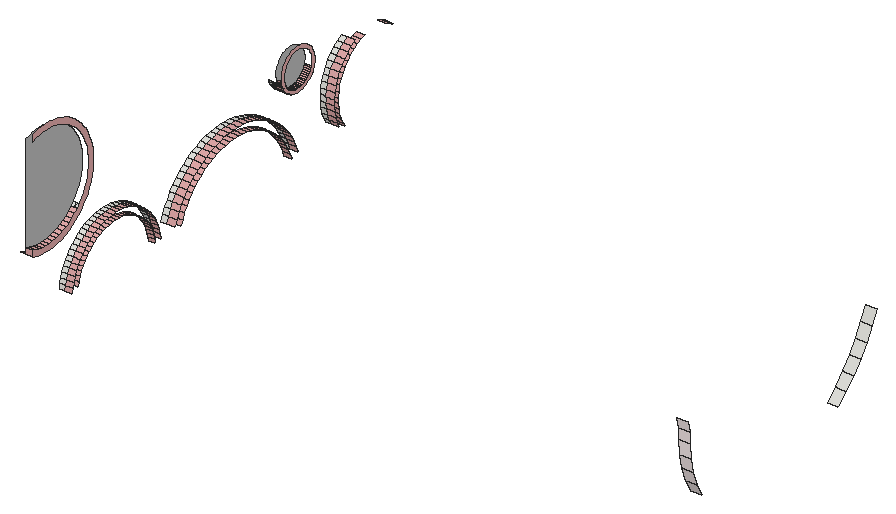
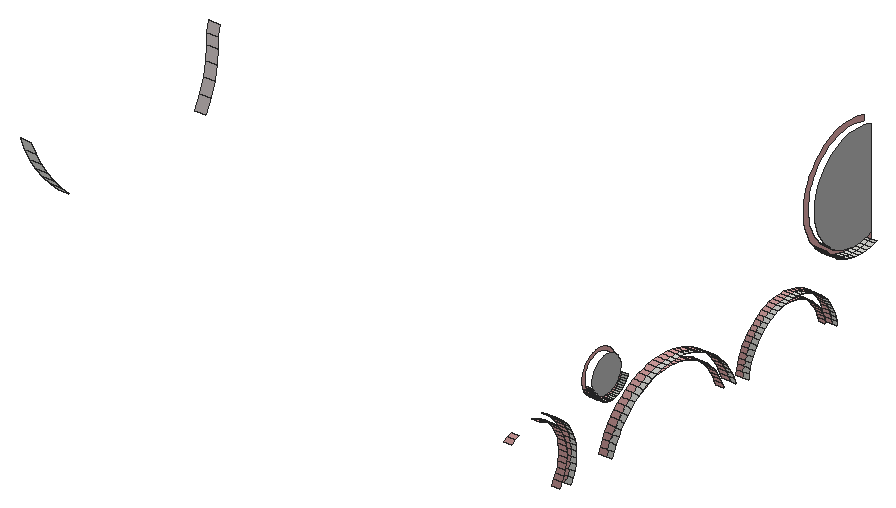
# SketchUp Ruby script. Lengths in inches.
U = 1.inch
M = Sketchup.active_model
def pt(a) = Geom::Point3d.new(a.map { |v| v * U })
def face(e, loops, mat)
  f = e.add_face(loops[0].map { |a| pt(a) })
  loops[1..].each { |l| e.add_face(l.map { |a| pt(a) }).erase! }
  f.material = f.back_material = mat if mat
  f
end
# faces: each face lists its corners as indices into pts; further lists are holes
def faces(e, pts, list, mat = nil) = list.each { |f| face(e, (f[0].is_a?(Array) ? f : [f]).map { |l| l.map { |i| pts[i] } }, mat) }
# xy, xz, yz: faces in a plane at the given z, y or x. An outline is a flat list of corners, or four numbers for a rectangle; further outlines are holes
def ring(l) = l.size == 4 ? [[l[0], l[1]], [l[2], l[1]], [l[2], l[3]], [l[0], l[3]]] : l.each_slice(2).to_a
def flat(e, list, mat, &to3) = list.each { |f| face(e, (f[0].is_a?(Array) ? f : [f]).map { |l| ring(l).map { |u, v| to3.(u, v) } }, mat) }
def xy(e, z, list, mat = nil) = flat(e, list, mat) { |x, y| [x, y, z] }
def xz(e, y, list, mat = nil) = flat(e, list, mat) { |x, z| [x, y, z] }
def yz(e, x, list, mat = nil) = flat(e, list, mat) { |y, z| [x, y, z] }
def lines(e, pts, list) = list.each { |a, b| e.add_line(pt(pts[a]), pt(pts[b])) }
# prism: a flat outline (further loops are holes) pulled along v
def prism(e, loops, v, mat = nil)
  f = face(e, loops, mat); d = Geom::Vector3d.new(v.map { |x| x * U })
  f.pushpull(f.normal.samedirection?(d) ? d.length : -d.length)
end
def box(e, o, s, mat = nil) = prism(e, [[o, [o[0] + s[0], o[1], o[2]], [o[0] + s[0], o[1] + s[1], o[2]], [o[0], o[1] + s[1], o[2]]]], [0, 0, s[2]], mat)
def at(x, y, z, deg = 0) = Geom::Transformation.translation(pt([x, y, z])) * Geom::Transformation.rotation(ORIGIN, Z_AXIS, deg.degrees)
def axes(o, x, y, z) = Geom::Transformation.new([*x, 0, *y, 0, *z, 0, *pt(o).to_a, 1])
def part(name) = M.definitions.add(name)
# library, detail: a bought-in or finely detailed component or shape, given as its bounding box
def library(name, o, s) = part(name).tap { |d| box(d.entities, o, s) }
def detail(e, o, s) = box(e.add_group.entities, o, s)
def put(e, d, t, mat = nil) = e.add_instance(d, t).tap { |i| i.material = mat if mat }
def group(e, t, mat = nil) = e.add_group.tap { |g| g.transformation = t; g.material = mat if mat }.entities
root = M.entities
M.materials.add("Generic").color = [224, 169, 169]
M.materials.add("Generic\#2").color = [246, 234, 234]
M.materials.add("[Mirror 01]").color = [185, 185, 185]
xy(root,79.24,[[10.6875,73.31,12.9375,74.91]],"Generic")
xz(root,0.4375,[[10.6875,80.35,12.625,82.1]],"Generic")
xz(root,109.61,[[9,71.81,10.6875,73.48]])
xz(root,109.61,[[10.6875,71.81,12.9375,73.48]],"Generic")
xz(root,111.05,[[10.6875,71.89,12.9375,73.4]],"Generic")
yz(root,10.6875,[[5.35,81.05,6.61,81.08,7.87,81.21,9.11,81.45,10.33,81.79,11.51,82.23,12.66,82.77,13.75,83.4,14.79,84.13,15.77,84.93,16.67,85.82,17.5,86.78,18.24,87.8,18.9,88.88,19.46,90.01,19.92,91.19,20.29,92.4,20.56,93.64,20.71,94.89,20.77,96.16,20.72,97.42,20.56,98.68,20.3,99.91,19.94,101.125,19.47,102.3,18.91,103.44,18.26,104.52,17.52,105.54,16.69,106.5,15.79,107.39,14.82,108.2,13.78,108.92,12.6875,109.56,11.54,110.1,10.36,110.54,9.14,110.89,7.9,111.13,6.64,111.26,5.38,111.29,4.11,111.22,2.86,111.04,1.63,110.75,0.4375,110.34,0.4375,82.1,1.6,81.6,2.83,81.3125,4.08,81.13],[96.45,81.98,96.96,82,97.45,82.06,97.94,82.17,98.42,82.33,98.875,82.53,99.3125,82.78,99.72,83.0625,100.1,83.39,100.45,83.75,100.76,84.14,101.04,84.5625,101.27,85.01,101.45,85.47,101.59,85.95,101.6875,86.45,101.73,86.95,101.73,87.45,101.68,87.95,101.58,88.4375,101.43,88.92,101.24,89.38,101.01,89.82,100.73,90.24,100.41,90.63,100.0625,90.99,99.68,91.31,99.26,91.59,98.82,91.83,98.36,92.03,97.89,92.18,97.4,92.29,96.9,92.34,96.4,92.35,95.9,92.3125,95.4,92.23,94.92,92.09,94.45,91.91,94,91.6875,93.58,91.42,93.18,91.11,92.82,90.77,92.49,90.39,92.2,89.99,91.94,89.55,91.74,89.1,91.57,88.625,91.45,88.14,91.39,87.64,91.36,87.14,91.39,86.64,91.47,86.14,91.59,85.66,91.76,85.18,91.97,84.73,92.23,84.3,92.52,83.9,92.86,83.52,93.23,83.18,93.63,82.88,94.06,82.62,94.51,82.4,94.98,82.23,95.46,82.1,95.95,82.01]],"[Mirror 01]")
yz(root,12.625,[[5.3125,79.45,6.71,79.48,8.1,79.625,9.48,79.89,10.83,80.27,12.14,80.75,13.4,81.35,14.61,82.05,15.76,82.85,16.84,83.74,17.84,84.72,18.75,85.78,19.58,86.91,20.3,88.11,20.92,89.36,21.44,90.66,21.84,92,22.14,93.37,22.3125,94.76,22.375,96.15,22.32,97.55,22.14,98.94,21.85,100.31,21.45,101.65,20.9375,102.95,20.32,104.21,19.6,105.4,18.78,106.54,17.86,107.6,16.87,108.58,15.79,109.47,14.64,110.28,13.43,110.98,12.17,111.58,10.86,112.07,9.51,112.45,8.14,112.71,6.75,112.87,5.35,112.9,3.95,112.82,2.57,112.62,1.18,112.3,0.4375,112.04,0.4375,110.34,1.63,110.75,2.86,111.04,4.11,111.22,5.38,111.29,6.64,111.26,7.9,111.13,9.14,110.89,10.36,110.54,11.54,110.1,12.6875,109.56,13.78,108.92,14.82,108.2,15.79,107.39,16.69,106.5,17.52,105.54,18.26,104.52,18.91,103.44,19.47,102.3,19.94,101.125,20.3,99.91,20.56,98.68,20.72,97.42,20.77,96.16,20.71,94.89,20.56,93.64,20.29,92.4,19.92,91.19,19.46,90.01,18.9,88.88,18.24,87.8,17.5,86.78,16.67,85.82,15.77,84.93,14.79,84.13,13.75,83.4,12.66,82.77,11.51,82.23,10.33,81.79,9.11,81.45,7.87,81.21,6.61,81.08,5.35,81.05,4.08,81.13,2.83,81.3125,1.6,81.6,0.4375,82.1,0.4375,80.35,1.09,80.07,2.53,79.73,3.92,79.53]],"Generic")
yz(root,12.9375,[[[96.4375,81.13,97.02,81.15,97.6,81.23,98.17,81.35,98.72,81.54,99.26,81.77,99.76,82.06,100.24,82.39,100.68,82.77,101.09,83.19,101.45,83.65,101.77,84.14,102.04,84.66,102.25,85.2,102.42,85.76,102.53,86.33,102.58,86.91,102.58,87.49,102.52,88.07,102.4,88.64,102.23,89.2,102.01,89.74,101.73,90.26,101.41,90.74,101.04,91.19,100.64,91.61,100.1875,91.98,99.71,92.3125,99.19,92.59,98.66,92.82,98.1,93,97.53,93.12,96.95,93.1875,96.37,93.2,95.79,93.15,95.22,93.05,94.65,92.9,94.11,92.6875,93.59,92.42,93.1,92.11,92.63,91.76,92.21,91.36,91.83,90.92,91.49,90.45,91.19,89.94,90.95,89.41,90.76,88.86,90.625,88.29,90.54,87.72,90.52,87.13,90.55,86.55,90.64,85.98,90.78,85.41,90.98,84.86,91.22,84.33,91.52,83.83,91.87,83.36,92.26,82.93,92.6875,82.53,93.15,82.18,93.65,81.88,94.17,81.62,94.72,81.42,95.28,81.27,95.86,81.17],[96.45,81.98,95.95,82.01,95.46,82.1,94.98,82.23,94.51,82.4,94.06,82.62,93.63,82.88,93.23,83.18,92.86,83.52,92.52,83.9,92.23,84.3,91.97,84.73,91.76,85.18,91.59,85.66,91.47,86.14,91.39,86.64,91.36,87.14,91.39,87.64,91.45,88.14,91.57,88.625,91.74,89.1,91.94,89.55,92.2,89.99,92.49,90.39,92.82,90.77,93.18,91.11,93.58,91.42,94,91.6875,94.45,91.91,94.92,92.09,95.4,92.23,95.9,92.3125,96.4,92.35,96.9,92.34,97.4,92.29,97.89,92.18,98.36,92.03,98.82,91.83,99.26,91.59,99.68,91.31,100.0625,90.99,100.41,90.63,100.73,90.24,101.01,89.82,101.24,89.38,101.43,88.92,101.58,88.4375,101.68,87.95,101.73,87.45,101.73,86.95,101.6875,86.45,101.59,85.95,101.45,85.47,101.27,85.01,101.04,84.5625,100.76,84.14,100.45,83.75,100.1,83.39,99.72,83.0625,99.3125,82.78,98.875,82.53,98.42,82.33,97.94,82.17,97.45,82.06,96.96,82]]],"Generic")
p = [[10.6875,44.75,65.51],[10.6875,44.96,64.32],[12.625,44.96,64.32],[12.625,44.75,65.51],[10.6875,14.89,65.81],[10.6875,14.66,64.44],
  [9,14.66,64.44],[9,14.89,65.81],[12.625,14.66,64.44],[12.625,14.89,65.81],[10.6875,46.99,64.59],[10.6875,46.75,65.95],
  [9,46.75,65.95],[9,46.99,64.59],[12.625,46.75,65.95],[12.625,46.99,64.59],[10.6875,53.89,64.92],[10.6875,54.48,66.42],
  [12.9375,54.48,66.42],[12.9375,53.89,64.92],[10.6875,93.7,66.35],[10.6875,94.28,64.86],[12.9375,94.28,64.86],[12.9375,93.7,66.35],
  [10.6875,113.5625,64.9],[10.6875,112.75,66.16],[12.9375,112.75,66.16],[12.9375,113.5625,64.9],[10.6875,16.89,65.39],[10.6875,17.1875,66.56],
  [12.625,17.1875,66.56],[12.625,16.89,65.39],[10.6875,110.75,66.95],[10.6875,111.49,65.45],[9,111.49,65.45],[9,110.75,66.95],
  [12.9375,111.49,65.45],[12.9375,110.75,66.95],[10.6875,44.4375,66.68],[12.625,44.4375,66.68],[184.0625,29.64,65.65],[184.0625,27.64,69.17],
  [180.9375,27.64,69.17],[180.9375,29.64,65.65],[10.6875,96.53,65.64],[10.6875,95.89,67.3],[9,95.89,67.3],[9,96.53,65.64],
  [12.9375,95.89,67.3],[12.9375,96.53,65.64],[10.6875,52.29,67.37],[10.6875,51.64,65.71],[9,51.64,65.71],[9,52.29,67.37],
  [12.9375,51.64,65.71],[12.9375,52.29,67.37],[10.6875,15.23,67.15],[9,15.23,67.15],[12.625,15.23,67.15],[10.6875,46.39,67.29],
  [9,46.39,67.29],[12.625,46.39,67.29],[10.6875,112.08,67.51],[12.9375,112.08,67.51],[10.6875,55.17,67.86],[12.9375,55.17,67.86],
  [10.6875,93.01,67.8],[12.9375,93.01,67.8],[10.6875,17.59,67.7],[12.625,17.59,67.7],[10.6875,44.03,67.82],[12.625,44.03,67.82],
  [184.0625,82.09,69.57],[184.0625,79.1875,66.78],[180.9375,79.1875,66.78],[180.9375,82.09,69.57],[10.6875,110.1875,68.52],[9,110.1875,68.52],
  [12.9375,110.1875,68.52],[10.6875,15.68,68.45],[9,15.68,68.45],[12.625,15.68,68.45],[10.6875,45.93,68.59],[9,45.93,68.59],
  [12.625,45.93,68.59],[10.6875,95.125,68.91],[9,95.125,68.91],[12.9375,95.125,68.91],[10.6875,53.06,68.97],[9,53.06,68.97],
  [12.9375,53.06,68.97],[10.6875,111.57,68.93],[12.9375,111.57,68.93],[10.6875,18.08,68.8],[12.625,18.08,68.8],[10.6875,43.53,68.92],
  [12.625,43.53,68.92],[10.6875,92.21,69.1875],[12.9375,92.21,69.1875],[10.6875,55.97,69.25],[12.9375,55.97,69.25],[10.6875,16.25,69.72],
  [9,16.25,69.72],[12.625,16.25,69.72],[10.6875,109.8,70.15],[9,109.8,70.15],[12.9375,109.8,70.15],[10.6875,45.35,69.85],
  [9,45.35,69.85],[12.625,45.35,69.85],[10.6875,18.66,69.86],[12.625,18.66,69.86],[10.6875,42.93,69.97],[12.625,42.93,69.97],
  [10.6875,94.24,70.45],[9,94.24,70.45],[12.9375,94.24,70.45],[10.6875,111.23,70.39],[12.9375,111.23,70.39],[10.6875,53.95,70.52],
  [9,53.95,70.52],[12.9375,53.95,70.52],[184.0625,26.21,72.96],[180.9375,26.21,72.96],[10.6875,56.87,70.57],[12.9375,56.87,70.57],
  [10.6875,91.32,70.51],[12.9375,91.32,70.51],[184.0625,84.78,72.57],[180.9375,84.78,72.57],[10.6875,16.92,70.93],[9,16.92,70.93],
  [12.625,16.92,70.93],[10.6875,44.67,71.05],[9,44.67,71.05],[12.625,44.67,71.05],[10.6875,19.34,70.87],[12.625,19.34,70.87],
  [10.6875,42.25,70.97],[12.625,42.25,70.97],[10.6875,109.61,71.81],[9,109.61,71.81],[12.9375,109.61,71.81],[10.6875,111.05,71.89],
  [12.9375,111.05,71.89],[10.6875,54.95,71.99],[9,54.95,71.99],[12.9375,54.95,71.99],[10.6875,90.32,71.77],[12.9375,90.32,71.77],
  [10.6875,93.24,71.92],[9,93.24,71.92],[12.9375,93.24,71.92],[10.6875,57.87,71.82],[12.9375,57.87,71.82],[10.6875,17.6875,72.08],
  [9,17.6875,72.08],[12.625,17.6875,72.08],[10.6875,20.09,71.8125],[12.625,20.09,71.8125],[10.6875,41.49,71.91],[12.625,41.49,71.91],
  [10.6875,43.89,72.19],[9,43.89,72.19],[12.625,43.89,72.19],[10.6875,20.93,72.69],[12.625,20.93,72.69],[10.6875,58.96,73],
  [12.9375,58.96,73],[10.6875,89.24,72.95],[12.9375,89.24,72.95],[10.6875,40.65,72.78],[12.625,40.65,72.78],[10.6875,92.14,73.32],
  [9,92.14,73.32],[12.9375,92.14,73.32],[10.6875,56.0625,73.38],[9,56.0625,73.38],[12.9375,56.0625,73.38],[10.6875,18.55,73.16],
  [9,18.55,73.16],[12.625,18.55,73.16],[10.6875,43.02,73.27],[9,43.02,73.27],[12.625,43.02,73.27],[184.0625,87.23,75.77],
  [180.9375,87.23,75.77],[10.6875,21.83,73.49],[12.625,21.83,73.49],[10.6875,39.73,73.57],[12.625,39.73,73.57],[10.6875,88.07,74.04],
  [12.9375,88.07,74.04],[184.0625,25.39,76.92],[180.9375,25.39,76.92],[10.6875,60.13,74.09],[12.9375,60.13,74.09],[10.6875,19.5,74.16],
  [9,19.5,74.16],[12.625,19.5,74.16],[10.6875,42.06,74.26],[9,42.06,74.26],[12.625,42.06,74.26],[10.6875,90.93,74.63],
  [9,90.93,74.63],[12.9375,90.93,74.63],[10.6875,57.27,74.68],[9,57.27,74.68],[12.9375,57.27,74.68],[10.6875,111.05,73.4],
  [10.6875,111.22,74.89],[12.9375,111.22,74.89],[12.9375,111.05,73.4],[10.6875,22.8,74.22],[12.625,22.8,74.22],[10.6875,109.8,75.14],
  [10.6875,109.61,73.48],[9,109.61,73.48],[9,109.8,75.14],[12.9375,109.61,73.48],[12.9375,109.8,75.14],[10.6875,38.76,74.29],
  [12.625,38.76,74.29],[10.6875,86.82,75.04],[12.9375,86.82,75.04],[10.6875,61.39,75.08],[12.9375,61.39,75.08],[10.6875,20.54,75.08],
  [9,20.54,75.08],[12.625,20.54,75.08],[10.6875,23.83,74.86],[12.625,23.83,74.86],[10.6875,37.73,74.92],[12.625,37.73,74.92],
  [10.6875,41.01,75.17],[9,41.01,75.17],[12.625,41.01,75.17],[10.6875,89.63,75.84],[9,89.63,75.84],[12.9375,89.63,75.84],
  [10.6875,58.58,75.89],[9,58.58,75.89],[12.9375,58.58,75.89],[10.6875,24.9,75.4],[12.625,24.9,75.4],[10.6875,36.64,75.46],
  [12.625,36.64,75.46],[10.6875,111.56,76.36],[12.9375,111.56,76.36],[10.6875,85.5,75.95],[12.9375,85.5,75.95],[10.6875,21.65,75.91],
  [9,21.65,75.91],[12.625,21.65,75.91],[10.6875,62.71,75.99],[12.9375,62.71,75.99],[10.6875,110.17,76.76],[9,110.17,76.76],
  [12.9375,110.17,76.76],[10.6875,39.9,75.99],[9,39.9,75.99],[12.625,39.9,75.99],[10.6875,26.03,75.86],[12.625,26.03,75.86],
  [10.6875,35.52,75.9],[12.625,35.52,75.9],[184.0625,89.4375,79.15],[180.9375,89.4375,79.15],[10.6875,88.24,76.96],[9,88.24,76.96],
  [12.9375,88.24,76.96],[10.6875,22.82,76.64],[9,22.82,76.64],[12.625,22.82,76.64],[10.6875,27.18,76.22],[12.625,27.18,76.22],
  [10.6875,34.36,76.25],[12.625,34.36,76.25],[10.6875,59.97,77],[9,59.97,77],[12.9375,59.97,77],[10.6875,84.11,76.75],
  [12.9375,84.11,76.75],[10.6875,38.72,76.71],[9,38.72,76.71],[12.625,38.72,76.71],[10.6875,64.1,76.79],[12.9375,64.1,76.79],
  [10.6875,28.36,76.48],[12.625,28.36,76.48],[10.6875,33.18,76.5],[12.625,33.18,76.5],[10.6875,112.0625,77.78],[12.9375,112.0625,77.78],
  [10.6875,29.56,76.64],[12.625,29.56,76.64],[10.6875,31.98,76.65],[12.625,31.98,76.65],[10.6875,24.05,77.26],[9,24.05,77.26],
  [12.625,24.05,77.26],[10.6875,30.77,76.7],[12.625,30.77,76.7],[10.6875,37.48,77.32],[9,37.48,77.32],[12.625,37.48,77.32],
  [10.6875,65.54,77.48],[12.9375,65.54,77.48],[10.6875,82.67,77.45],[12.9375,82.67,77.45],[10.6875,110.73,78.34],[9,110.73,78.34],
  [12.9375,110.73,78.34],[184.0625,25.2,80.97],[180.9375,25.2,80.97],[10.6875,61.44,78.01],[9,61.44,78.01],[12.9375,61.44,78.01],
  [10.6875,86.77,77.97],[9,86.77,77.97],[12.9375,86.77,77.97],[10.6875,25.34,77.79],[9,25.34,77.79],[12.625,25.34,77.79],
  [10.6875,36.19,77.83],[9,36.19,77.83],[12.625,36.19,77.83],[10.6875,67.03,78.0625],[12.9375,67.03,78.0625],[10.6875,81.18,78.04],
  [12.9375,81.18,78.04],[10.6875,26.66,78.2],[9,26.66,78.2],[12.625,26.66,78.2],[10.6875,34.87,78.23],[9,34.87,78.23],
  [12.625,34.87,78.23],[10.6875,112.73,79.13],[12.9375,112.73,79.13],[10.6875,62.98,78.9],[9,62.98,78.9],[12.9375,62.98,78.9],
  [10.6875,79.65,78.52],[12.9375,79.65,78.52],[10.6875,85.23,78.86],[9,85.23,78.86],[12.9375,85.23,78.86],[10.6875,68.5625,78.53],
  [12.9375,68.5625,78.53],[10.6875,28.01,78.49],[9,28.01,78.49],[12.625,28.01,78.49],[10.6875,33.51,78.52],[9,33.51,78.52],
  [12.625,33.51,78.52],[10.6875,111.47,79.84],[9,111.47,79.84],[12.9375,111.47,79.84],[10.6875,29.38,78.68],[9,29.38,78.68],
  [12.625,29.38,78.68],[10.6875,32.14,78.6875],[9,32.14,78.6875],[12.625,32.14,78.6875],[10.6875,70.125,78.89],[12.9375,70.125,78.89],
  [10.6875,78.09,78.875],[12.9375,78.09,78.875],[10.6875,30.76,78.74],[9,30.76,78.74],[12.625,30.76,78.74],[10.6875,64.59,79.67],
  [9,64.59,79.67],[12.9375,64.59,79.67],[10.6875,71.71,79.125],[12.9375,71.71,79.125],[10.6875,76.51,79.12],[12.9375,76.51,79.12],
  [10.6875,83.63,79.64],[9,83.63,79.64],[12.9375,83.63,79.64],[10.6875,73.31,79.24],[12.9375,73.31,79.24],[10.6875,74.91,79.24],
  [12.9375,74.91,79.24],[184.0625,91.38,82.68],[180.9375,91.38,82.68],[10.6875,113.54,80.4],[12.9375,113.54,80.4],[10.6875,3.92,79.53],
  [10.6875,5.3125,79.45],[9,5.3125,79.45],[9,3.92,79.53],[12.625,5.3125,79.45],[12.625,3.92,79.53],[10.6875,6.71,79.48],
  [9,6.71,79.48],[12.625,6.71,79.48],[10.6875,2.53,79.73],[9,2.53,79.73],[12.625,2.53,79.73],[10.6875,8.1,79.625],
  [9,8.1,79.625],[12.625,8.1,79.625],[10.6875,9.48,79.89],[9,9.48,79.89],[12.625,9.48,79.89],[10.6875,81.97,80.29],
  [9,81.97,80.29],[12.9375,81.97,80.29],[10.6875,1.09,80.07],[9,1.09,80.07],[12.625,1.09,80.07],[10.6875,66.25,80.32],
  [9,66.25,80.32],[12.9375,66.25,80.32],[10.6875,112.37,81.25],[9,112.37,81.25],[12.9375,112.37,81.25],[10.6875,10.83,80.27],
  [9,10.83,80.27],[12.625,10.83,80.27],[10.6875,0.4375,80.35],[9,0.4375,80.35],[12.625,0.4375,80.35],[10.6875,12.14,80.75],
  [9,12.14,80.75],[12.625,12.14,80.75],[10.6875,67.95,80.84],[9,67.95,80.84],[12.9375,67.95,80.84],[10.6875,80.27,80.82],
  [9,80.27,80.82],[12.9375,80.27,80.82],[10.6875,114.49,81.57],[12.9375,114.49,81.57],[10.6875,13.4,81.35],[9,13.4,81.35],
  [12.625,13.4,81.35],[10.6875,69.69,81.23],[9,69.69,81.23],[12.9375,69.69,81.23],[10.6875,78.54,81.22],[9,78.54,81.22],
  [12.9375,78.54,81.22],[184.0625,25.04,84],[180.9375,25.04,84],[10.6875,4.08,81.13],[10.6875,2.83,81.3125],[12.625,2.83,81.3125],
  [12.625,4.08,81.13],[10.6875,5.35,81.05],[12.625,5.35,81.05],[10.6875,6.61,81.08],[12.625,6.61,81.08],[10.6875,7.87,81.21],
  [12.625,7.87,81.21],[10.6875,95.86,81.17],[10.6875,96.4375,81.13],[9,96.4375,81.13],[9,95.86,81.17],[12.9375,96.4375,81.13],
  [12.9375,95.86,81.17],[10.6875,97.02,81.15],[9,97.02,81.15],[12.9375,97.02,81.15],[10.6875,9.11,81.45],[12.625,9.11,81.45],
  [10.6875,71.45,81.5],[9,71.45,81.5],[12.9375,71.45,81.5],[10.6875,76.78,81.49],[9,76.78,81.49],[12.9375,76.78,81.49],
  [10.6875,95.28,81.27],[9,95.28,81.27],[12.9375,95.28,81.27],[10.6875,97.6,81.23],[9,97.6,81.23],[12.9375,97.6,81.23],
  [10.6875,98.17,81.35],[9,98.17,81.35],[12.9375,98.17,81.35],[10.6875,113.42,82.54],[9,113.42,82.54],[12.9375,113.42,82.54],
  [10.6875,1.6,81.6],[12.625,1.6,81.6],[10.6875,94.72,81.42],[9,94.72,81.42],[12.9375,94.72,81.42],[10.6875,10.33,81.79],
  [12.625,10.33,81.79],[10.6875,14.61,82.05],[9,14.61,82.05],[12.625,14.61,82.05],[10.6875,94.17,81.62],[9,94.17,81.62],
  [12.9375,94.17,81.62],[10.6875,98.72,81.54],[9,98.72,81.54],[12.9375,98.72,81.54],[10.6875,73.22,81.63],[9,73.22,81.63],
  [12.9375,73.22,81.63],[10.6875,75,81.625],[9,75,81.625],[12.9375,75,81.625],[10.6875,99.26,81.77],[9,99.26,81.77],
  [12.9375,99.26,81.77],[10.6875,0.4375,82.1],[12.625,0.4375,82.1],[10.6875,93.65,81.88],[9,93.65,81.88],[12.9375,93.65,81.88],
  [10.6875,115.57,82.62],[12.9375,115.57,82.62],[10.6875,11.51,82.23],[12.625,11.51,82.23],[10.6875,99.76,82.06],[9,99.76,82.06],
  [12.9375,99.76,82.06],[10.6875,93.15,82.18],[9,93.15,82.18],[12.9375,93.15,82.18],[10.6875,95.95,82.01],[10.6875,95.46,82.1],
  [12.9375,95.46,82.1],[12.9375,95.95,82.01],[10.6875,96.45,81.98],[12.9375,96.45,81.98],[10.6875,96.96,82],[12.9375,96.96,82],
  [10.6875,97.45,82.06],[12.9375,97.45,82.06],[10.6875,15.76,82.85],[9,15.76,82.85],[12.625,15.76,82.85],[10.6875,94.98,82.23],
  [12.9375,94.98,82.23],[10.6875,97.94,82.17],[12.9375,97.94,82.17],[10.6875,100.24,82.39],[9,100.24,82.39],[12.9375,100.24,82.39],
  [10.6875,12.66,82.77],[12.625,12.66,82.77],[10.6875,92.6875,82.53],[9,92.6875,82.53],[12.9375,92.6875,82.53],[10.6875,94.51,82.4],
  [12.9375,94.51,82.4],[10.6875,98.42,82.33],[12.9375,98.42,82.33],[10.6875,98.875,82.53],[12.9375,98.875,82.53],[10.6875,94.06,82.62],
  [12.9375,94.06,82.62],[10.6875,100.68,82.77],[9,100.68,82.77],[12.9375,100.68,82.77],[10.6875,92.26,82.93],[9,92.26,82.93],
  [12.9375,92.26,82.93],[10.6875,99.3125,82.78],[12.9375,99.3125,82.78],[10.6875,114.62,83.71],[9,114.62,83.71],[12.9375,114.62,83.71],
  [10.6875,93.63,82.88],[12.9375,93.63,82.88],[10.6875,116.76,83.54],[12.9375,116.76,83.54],[184.0625,93.05,86.35],[180.9375,93.05,86.35],
  [10.6875,13.75,83.4],[12.625,13.75,83.4],[10.6875,16.84,83.74],[9,16.84,83.74],[12.625,16.84,83.74],[10.6875,99.72,83.0625],
  [12.9375,99.72,83.0625],[10.6875,101.09,83.19],[9,101.09,83.19],[12.9375,101.09,83.19],[10.6875,91.87,83.36],[9,91.87,83.36],
  [12.9375,91.87,83.36],[10.6875,93.23,83.18],[12.9375,93.23,83.18],[10.6875,100.1,83.39],[12.9375,100.1,83.39],[10.6875,92.86,83.52],
  [12.9375,92.86,83.52],[10.6875,101.45,83.65],[9,101.45,83.65],[12.9375,101.45,83.65],[10.6875,14.79,84.13],[12.625,14.79,84.13],
  [10.6875,91.52,83.83],[9,91.52,83.83],[12.9375,91.52,83.83],[10.6875,100.45,83.75],[12.9375,100.45,83.75],[10.6875,92.52,83.9],
  [12.9375,92.52,83.9],[10.6875,118.05,84.32],[12.9375,118.05,84.32],[10.6875,101.77,84.14],[9,101.77,84.14],[12.9375,101.77,84.14],
  [10.6875,17.84,84.72],[9,17.84,84.72],[12.625,17.84,84.72],[10.6875,100.76,84.14],[12.9375,100.76,84.14],[10.6875,115.94,84.73],
  [9,115.94,84.73],[12.9375,115.94,84.73],[10.6875,91.22,84.33],[9,91.22,84.33],[12.9375,91.22,84.33],[10.6875,92.23,84.3],
  [12.9375,92.23,84.3],[184.0625,24.39,86.97],[180.9375,24.39,86.97],[10.6875,129.68,84.67],[10.6875,131.01,83.97],[12.9375,131.01,83.97],
  [12.9375,129.68,84.67],[10.6875,15.77,84.93],[12.625,15.77,84.93],[10.6875,101.04,84.5625],[12.9375,101.04,84.5625],[10.6875,102.04,84.66],
  [9,102.04,84.66],[12.9375,102.04,84.66],[10.6875,90.98,84.86],[9,90.98,84.86],[12.9375,90.98,84.86],[10.6875,91.97,84.73],
  [12.9375,91.97,84.73],[10.6875,119.41,84.95],[12.9375,119.41,84.95],[10.6875,101.27,85.01],[12.9375,101.27,85.01],[10.6875,18.75,85.78],
  [9,18.75,85.78],[12.625,18.75,85.78],[10.6875,91.76,85.18],[12.9375,91.76,85.18],[10.6875,102.25,85.2],[9,102.25,85.2],
  [12.9375,102.25,85.2],[10.6875,117.37,85.6],[9,117.37,85.6],[12.9375,117.37,85.6],[10.6875,128.27,85.21],[12.9375,128.27,85.21],
  [10.6875,16.67,85.82],[12.625,16.67,85.82],[10.6875,90.78,85.41],[9,90.78,85.41],[12.9375,90.78,85.41],[10.6875,120.85,85.41],
  [12.9375,120.85,85.41],[10.6875,101.45,85.47],[12.9375,101.45,85.47],[10.6875,91.59,85.66],[12.9375,91.59,85.66]]
faces(root,p,[[0,1,2,3],[4,5,8,9],[10,11,14,15],[16,17,18,19],[20,21,22,23],[24,25,26,27],[28,29,30,31],[32,33,36,37],
  [38,0,3,39],[44,45,48,49],[50,51,54,55],[56,4,9,58],[11,59,61,14],[25,62,63,26],[17,64,65,18],[66,20,23,67],
  [29,68,69,30],[70,38,39,71],[76,32,37,78],[79,56,58,81],[59,82,84,61],[45,85,87,48],[88,50,55,90],[62,91,92,63],
  [68,93,94,69],[95,70,71,96],[97,66,67,98],[64,99,100,65],[101,79,81,103],[104,76,78,106],[82,107,109,84],[93,110,111,94],
  [112,95,96,113],[85,114,116,87],[91,117,118,92],[119,88,90,121],[99,124,125,100],[126,97,98,127],[130,101,103,132],[107,133,135,109],
  [110,136,137,111],[138,112,113,139],[140,104,106,142],[117,143,144,118],[145,119,121,147],[148,126,127,149],[114,150,152,116],[124,153,154,125],
  [155,130,132,157],[136,158,159,137],[160,138,139,161],[133,162,164,135],[158,165,166,159],[153,167,168,154],[169,148,149,170],[171,160,161,172],
  [150,173,175,152],[176,145,147,178],[179,155,157,181],[162,182,184,164],[165,187,188,166],[189,171,172,190],[191,169,170,192],[167,195,196,168],
  [197,179,181,199],[182,200,202,184],[173,203,205,175],[206,176,178,208],[209,210,211,212],[187,213,214,188],[215,216,219,220],[221,189,190,222],
  [223,191,192,224],[195,225,226,196],[227,197,199,229],[213,230,231,214],[232,221,222,233],[200,234,236,202],[203,237,239,205],[240,206,208,242],
  [230,243,244,231],[245,232,233,246],[210,247,248,211],[249,223,224,250],[251,227,229,253],[225,254,255,226],[256,215,220,258],[234,259,261,236],
  [243,262,263,244],[264,245,246,265],[237,268,270,239],[271,251,253,273],[262,274,275,263],[276,264,265,277],[278,240,242,280],[281,249,250,282],
  [259,283,285,261],[254,286,287,255],[274,288,289,275],[290,276,277,291],[247,292,293,248],[288,294,295,289],[296,290,291,297],[298,271,273,300],
  [294,301,302,295],[301,296,297,302],[283,303,305,285],[286,306,307,287],[308,281,282,309],[310,256,258,312],[315,278,280,317],[268,318,320,270],
  [321,298,300,323],[303,324,326,305],[306,327,328,307],[329,308,309,330],[331,321,323,333],[324,334,336,326],[292,337,338,293],[339,315,317,341],
  [342,329,330,343],[318,344,346,320],[327,347,348,328],[349,331,333,351],[334,352,354,336],[355,310,312,357],[358,349,351,360],[352,361,363,354],
  [347,364,365,348],[366,342,343,367],[368,358,360,370],[361,368,370,363],[371,339,341,373],[364,374,375,365],[376,366,367,377],[344,378,380,346],
  [374,381,382,375],[383,376,377,384],[337,387,388,338],[378,407,409,380],[413,371,373,415],[416,355,357,418],[428,413,415,430],[407,431,433,409],
  [387,434,435,388],[439,428,430,441],[431,442,444,433],[447,448,449,450],[451,447,450,452],[453,451,452,454],[455,453,454,456],[457,458,461,462],
  [458,463,465,461],[466,455,456,467],[468,439,441,470],[442,471,473,444],[474,457,462,476],[463,477,479,465],[477,480,482,479],[483,416,418,485],
  [448,486,487,449],[488,474,476,490],[491,466,467,492],[496,488,490,498],[480,499,501,482],[502,468,470,504],[471,505,507,473],[499,508,510,501],
  [486,511,512,487],[505,502,504,507],[513,496,498,515],[434,516,517,435],[518,491,492,519],[508,520,522,510],[523,513,515,525],[526,527,528,529],
  [530,526,529,531],[532,530,531,533],[534,532,533,535],[527,539,540,528],[541,534,535,542],[520,543,545,522],[546,518,519,547],[548,523,525,550],
  [539,551,552,540],[553,541,542,554],[555,553,554,556],[551,557,558,552],[543,559,561,545],[562,548,550,564],[565,555,556,566],[567,483,485,569],
  [557,570,571,558],[516,572,573,517],[576,546,547,577],[581,565,566,582],[559,583,585,561],[586,562,564,588],[570,589,590,571],[591,581,582,592],
  [589,593,594,590],[583,595,597,585],[598,576,577,599],[600,586,588,602],[603,591,592,604],[593,605,606,594],[572,607,608,573],[595,609,611,597],
  [615,603,604,616],[617,567,569,619],[620,600,602,622],[605,623,624,606],[627,628,629,630],[631,598,599,632],[633,615,616,634],[609,635,637,611],
  [638,620,622,640],[623,641,642,624],[607,643,644,608],[645,633,634,646],[641,650,651,642],[635,652,654,637],[655,617,619,657],[658,627,630,659],
  [660,631,632,661],[662,638,640,664],[643,665,666,644],[667,645,646,668],[650,669,670,651]],"Generic")
faces(root,p,[[4,5,6,7],[10,11,12,13],[32,33,34,35],[44,45,46,47],[50,51,52,53],[56,4,7,57],[11,59,60,12],[72,73,74,75],
  [76,32,35,77],[79,56,57,80],[59,82,83,60],[45,85,86,46],[88,50,53,89],[101,79,80,102],[104,76,77,105],[82,107,108,83],
  [85,114,115,86],[119,88,89,120],[128,72,75,129],[130,101,102,131],[107,133,134,108],[140,104,105,141],[145,119,120,146],[114,150,151,115],
  [155,130,131,156],[133,162,163,134],[150,173,174,151],[176,145,146,177],[179,155,156,180],[162,182,183,163],[185,128,129,186],[197,179,180,198],
  [182,200,201,183],[173,203,204,174],[206,176,177,207],[215,216,217,218],[227,197,198,228],[200,234,235,201],[203,237,238,204],[240,206,207,241],
  [251,227,228,252],[256,215,218,257],[234,259,260,235],[266,185,186,267],[237,268,269,238],[271,251,252,272],[278,240,241,279],[259,283,284,260],
  [298,271,272,299],[283,303,304,284],[310,256,257,311],[315,278,279,316],[268,318,319,269],[321,298,299,322],[303,324,325,304],[331,321,322,332],
  [324,334,335,325],[339,315,316,340],[318,344,345,319],[349,331,332,350],[334,352,353,335],[355,310,311,356],[358,349,350,359],[352,361,362,353],
  [368,358,359,369],[361,368,369,362],[371,339,340,372],[344,378,379,345],[385,266,267,386],[389,390,391,392],[389,390,393,394],[390,395,396,391],
  [390,395,397,393],[398,389,392,399],[398,389,394,400],[395,401,402,396],[395,401,403,397],[401,404,405,402],[401,404,406,403],[378,407,408,379],
  [410,398,399,411],[410,398,400,412],[413,371,372,414],[416,355,356,417],[404,419,420,405],[404,419,421,406],[422,410,411,423],[422,410,412,424],
  [419,425,426,420],[419,425,427,421],[428,413,414,429],[407,431,432,408],[425,436,437,426],[425,436,438,427],[439,428,429,440],[431,442,443,432],
  [457,458,459,460],[458,463,464,459],[468,439,440,469],[442,471,472,443],[474,457,460,475],[463,477,478,464],[477,480,481,478],[483,416,417,484],
  [488,474,475,489],[436,493,494,437],[436,493,495,438],[496,488,489,497],[480,499,500,481],[502,468,469,503],[471,505,506,472],[499,508,509,500],
  [505,502,503,506],[513,496,497,514],[508,520,521,509],[523,513,514,524],[493,536,537,494],[493,536,538,495],[520,543,544,521],[548,523,524,549],
  [543,559,560,544],[562,548,549,563],[567,483,484,568],[574,385,386,575],[536,578,579,537],[536,578,580,538],[559,583,584,560],[586,562,563,587],
  [583,595,596,584],[600,586,587,601],[595,609,610,596],[578,612,613,579],[578,612,614,580],[617,567,568,618],[620,600,601,621],[609,635,636,610],
  [638,620,621,639],[612,647,648,613],[612,647,649,614],[635,652,653,636],[655,617,618,656],[662,638,639,663]])
faces(root,p,[[40,41,42,43],[41,122,123,42],[122,193,194,123],[193,313,314,194],[313,445,446,314],[445,625,626,446]],"Generic\#2")
